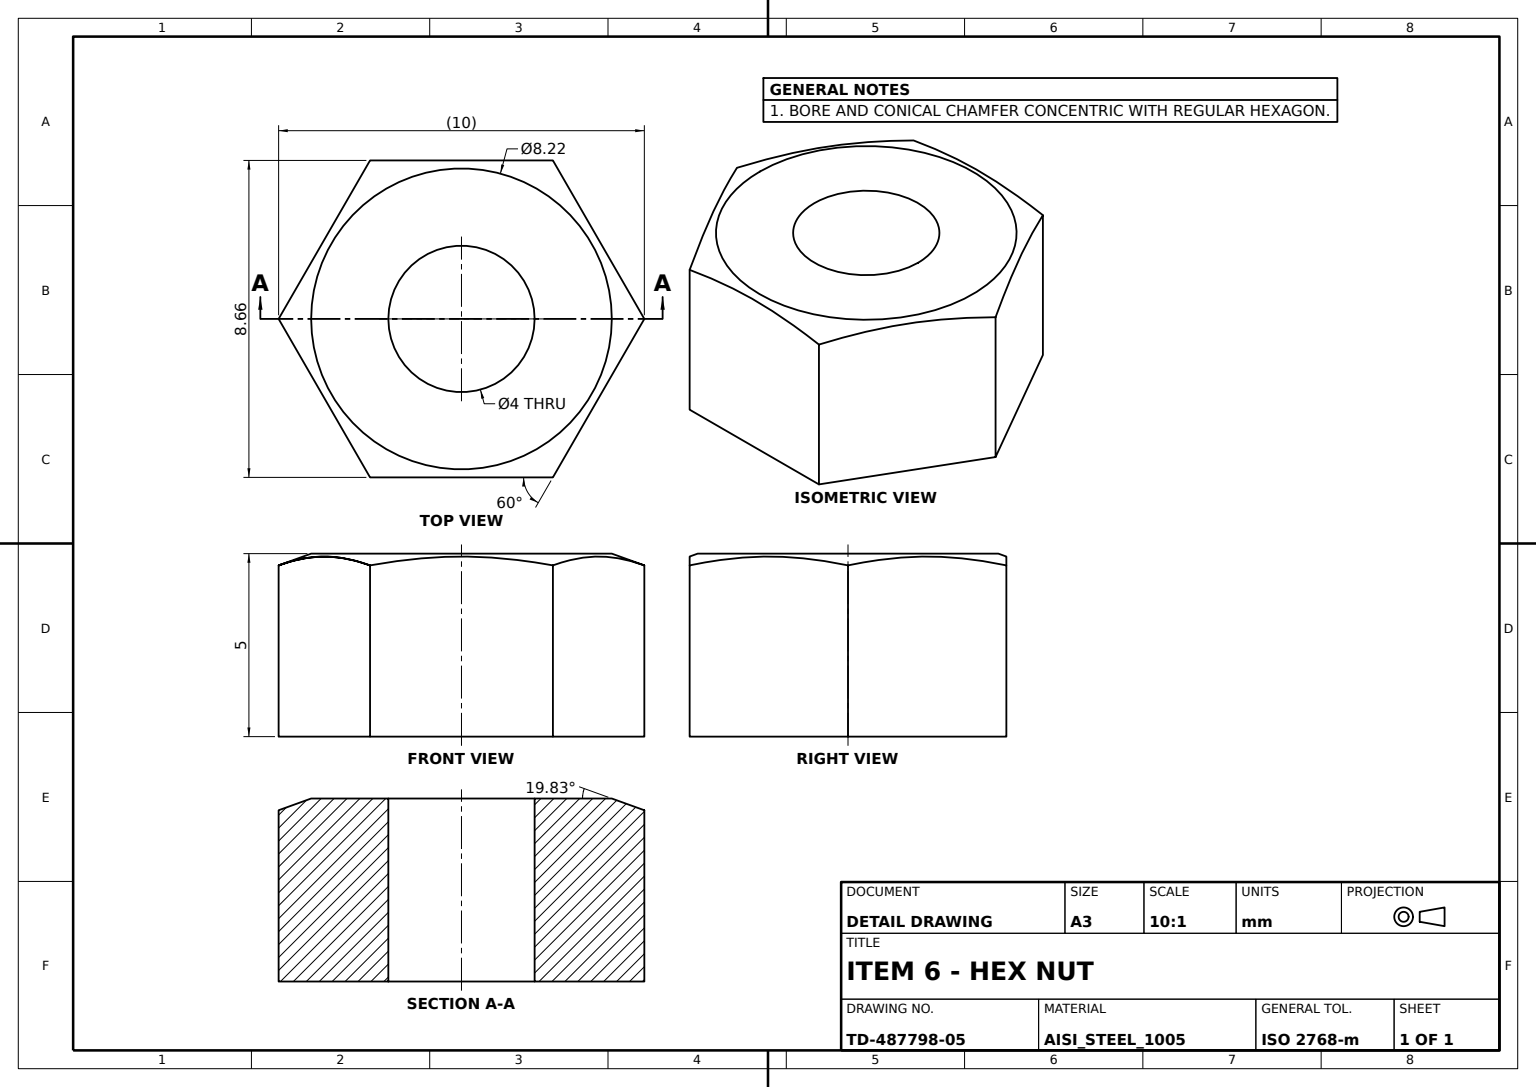
ISO-10303-21;
HEADER;
FILE_DESCRIPTION((''),'2;1');
FILE_NAME('','',(''),(''),'','','');
FILE_SCHEMA(('AUTOMOTIVE_DESIGN'));
ENDSEC;
DATA;
#1=APPLICATION_CONTEXT('');
#2=PRODUCT_CONTEXT('',#1,'mechanical');
#3=PRODUCT('','','',(#2));
#4=PRODUCT_DEFINITION_FORMATION('','',#3);
#5=PRODUCT_DEFINITION_CONTEXT('',#1,'design');
#6=PRODUCT_DEFINITION('','',#4,#5);
#7=PRODUCT_DEFINITION_SHAPE('','',#6);
#8=(LENGTH_UNIT()NAMED_UNIT(*)SI_UNIT(.MILLI.,.METRE.));
#9=(NAMED_UNIT(*)PLANE_ANGLE_UNIT()SI_UNIT($,.RADIAN.));
#10=(NAMED_UNIT(*)SI_UNIT($,.STERADIAN.)SOLID_ANGLE_UNIT());
#11=UNCERTAINTY_MEASURE_WITH_UNIT(LENGTH_MEASURE(0.005),#8,'distance_accuracy_value','');
#12=(GEOMETRIC_REPRESENTATION_CONTEXT(3)GLOBAL_UNCERTAINTY_ASSIGNED_CONTEXT((#11))GLOBAL_UNIT_ASSIGNED_CONTEXT((#8,#9,#10))REPRESENTATION_CONTEXT('',''));
#13=CARTESIAN_POINT('',(-2.5,-4.330127,4.679253));
#14=VERTEX_POINT('',#13);
#15=CARTESIAN_POINT('',(-5.,0.,4.679253));
#16=VERTEX_POINT('',#15);
#17=CARTESIAN_POINT('',(-2.916667,-3.608439,4.829483));
#18=CARTESIAN_POINT('',(-3.75,-2.165064,5.012071));
#19=CARTESIAN_POINT('',(-4.583333,-0.721688,4.829483));
#20=B_SPLINE_CURVE_WITH_KNOTS('',3,(#13,#17,#18,#19,#15),.UNSPECIFIED.,.F.,.F.,(4,1,4),(0.000000231,0.002500231,0.005000231),.UNSPECIFIED.);
#21=EDGE_CURVE('',#14,#16,#20,.T.);
#22=ORIENTED_EDGE('',*,*,#21,.T.);
#23=CARTESIAN_POINT('',(-5.,0.,0.));
#24=VERTEX_POINT('',#23);
#25=CARTESIAN_POINT('',(-5.,0.,5.));
#26=DIRECTION('',(0.,0.,-1.));
#27=VECTOR('',#26,1000.);
#28=LINE('',#25,#27);
#29=EDGE_CURVE('',#16,#24,#28,.T.);
#30=ORIENTED_EDGE('',*,*,#29,.T.);
#31=CARTESIAN_POINT('',(-2.5,-4.330127,0.));
#32=VERTEX_POINT('',#31);
#33=DIRECTION('',(0.5,-0.866025404,0.));
#34=VECTOR('',#33,1000.);
#35=LINE('',#23,#34);
#36=EDGE_CURVE('',#24,#32,#35,.T.);
#37=ORIENTED_EDGE('',*,*,#36,.T.);
#38=CARTESIAN_POINT('',(-2.5,-4.330127,5.));
#39=LINE('',#38,#27);
#40=EDGE_CURVE('',#14,#32,#39,.T.);
#41=ORIENTED_EDGE('',*,*,#40,.F.);
#42=EDGE_LOOP('',(#22,#30,#37,#41));
#43=FACE_BOUND('',#42,.T.);
#44=DIRECTION('',(0.866025404,0.5,0.));
#45=DIRECTION('',(-0.5,0.866025404,0.));
#46=AXIS2_PLACEMENT_3D('',#25,#44,#45);
#47=PLANE('',#46);
#48=ADVANCED_FACE('',(#43),#47,.F.);
#49=CARTESIAN_POINT('',(2.,0.,0.));
#50=VERTEX_POINT('',#49);
#51=CARTESIAN_POINT('',(0.,0.,0.));
#52=DIRECTION('',(1.,0.,0.));
#53=AXIS2_PLACEMENT_3D('',#51,#26,#52);
#54=CIRCLE('',#53,2.);
#55=EDGE_CURVE('',#50,#50,#54,.T.);
#56=ORIENTED_EDGE('',*,*,#55,.T.);
#57=EDGE_LOOP('',(#56));
#58=FACE_BOUND('',#57,.T.);
#59=CARTESIAN_POINT('',(2.,0.,5.));
#60=VERTEX_POINT('',#59);
#61=CARTESIAN_POINT('',(0.,0.,5.));
#62=AXIS2_PLACEMENT_3D('',#61,#26,#52);
#63=CIRCLE('',#62,2.);
#64=EDGE_CURVE('',#60,#60,#63,.T.);
#65=ORIENTED_EDGE('',*,*,#64,.F.);
#66=EDGE_LOOP('',(#65));
#67=FACE_BOUND('',#66,.T.);
#68=DIRECTION('',(0.,0.,1.));
#69=AXIS2_PLACEMENT_3D('',#51,#68,#52);
#70=CYLINDRICAL_SURFACE('',#69,2.);
#71=ADVANCED_FACE('',(#58,#67),#70,.F.);
#72=CARTESIAN_POINT('',(5.,0.,4.679253));
#73=VERTEX_POINT('',#72);
#74=CARTESIAN_POINT('',(5.,0.,0.));
#75=VERTEX_POINT('',#74);
#76=CARTESIAN_POINT('',(5.,0.,5.));
#77=LINE('',#76,#27);
#78=EDGE_CURVE('',#73,#75,#77,.T.);
#79=ORIENTED_EDGE('',*,*,#78,.F.);
#80=CARTESIAN_POINT('',(2.5,-4.330127,4.679253));
#81=VERTEX_POINT('',#80);
#82=CARTESIAN_POINT('',(4.583333,-0.721688,4.829483));
#83=CARTESIAN_POINT('',(3.75,-2.165064,5.012071));
#84=CARTESIAN_POINT('',(2.916667,-3.608439,4.829483));
#85=B_SPLINE_CURVE_WITH_KNOTS('',3,(#72,#82,#83,#84,#80),.UNSPECIFIED.,.F.,.F.,(4,1,4),(0.000000231,0.002500231,0.005000231),.UNSPECIFIED.);
#86=EDGE_CURVE('',#73,#81,#85,.T.);
#87=ORIENTED_EDGE('',*,*,#86,.T.);
#88=CARTESIAN_POINT('',(2.5,-4.330127,0.));
#89=VERTEX_POINT('',#88);
#90=CARTESIAN_POINT('',(2.5,-4.330127,5.));
#91=LINE('',#90,#27);
#92=EDGE_CURVE('',#81,#89,#91,.T.);
#93=ORIENTED_EDGE('',*,*,#92,.T.);
#94=DIRECTION('',(0.5,0.866025404,0.));
#95=VECTOR('',#94,1000.);
#96=LINE('',#88,#95);
#97=EDGE_CURVE('',#89,#75,#96,.T.);
#98=ORIENTED_EDGE('',*,*,#97,.T.);
#99=EDGE_LOOP('',(#79,#87,#93,#98));
#100=FACE_BOUND('',#99,.T.);
#101=DIRECTION('',(-0.866025404,0.5,0.));
#102=DIRECTION('',(-0.5,-0.866025404,0.));
#103=AXIS2_PLACEMENT_3D('',#90,#101,#102);
#104=PLANE('',#103);
#105=ADVANCED_FACE('',(#100),#104,.F.);
#106=CARTESIAN_POINT('',(2.5,4.330127,4.679253));
#107=VERTEX_POINT('',#106);
#108=CARTESIAN_POINT('',(2.916667,3.608439,4.829483));
#109=CARTESIAN_POINT('',(3.75,2.165064,5.012071));
#110=CARTESIAN_POINT('',(4.583333,0.721688,4.829483));
#111=B_SPLINE_CURVE_WITH_KNOTS('',3,(#106,#108,#109,#110,#72),.UNSPECIFIED.,.F.,.F.,(4,1,4),(0.000000231,0.002500231,0.005000231),.UNSPECIFIED.);
#112=EDGE_CURVE('',#107,#73,#111,.T.);
#113=ORIENTED_EDGE('',*,*,#112,.T.);
#114=ORIENTED_EDGE('',*,*,#78,.T.);
#115=CARTESIAN_POINT('',(2.5,4.330127,0.));
#116=VERTEX_POINT('',#115);
#117=VECTOR('',#45,1000.);
#118=LINE('',#74,#117);
#119=EDGE_CURVE('',#75,#116,#118,.T.);
#120=ORIENTED_EDGE('',*,*,#119,.T.);
#121=CARTESIAN_POINT('',(2.5,4.330127,5.));
#122=LINE('',#121,#27);
#123=EDGE_CURVE('',#107,#116,#122,.T.);
#124=ORIENTED_EDGE('',*,*,#123,.F.);
#125=EDGE_LOOP('',(#113,#114,#120,#124));
#126=FACE_BOUND('',#125,.T.);
#127=DIRECTION('',(-0.866025404,-0.5,0.));
#128=AXIS2_PLACEMENT_3D('',#76,#127,#33);
#129=PLANE('',#128);
#130=ADVANCED_FACE('',(#126),#129,.F.);
#131=ORIENTED_EDGE('',*,*,#29,.F.);
#132=CARTESIAN_POINT('',(-2.5,4.330127,4.679253));
#133=VERTEX_POINT('',#132);
#134=CARTESIAN_POINT('',(-4.583333,0.721688,4.829483));
#135=CARTESIAN_POINT('',(-3.75,2.165064,5.012071));
#136=CARTESIAN_POINT('',(-2.916667,3.608439,4.829483));
#137=B_SPLINE_CURVE_WITH_KNOTS('',3,(#15,#134,#135,#136,#132),.UNSPECIFIED.,.F.,.F.,(4,1,4),(0.000000231,0.002500231,0.005000231),.UNSPECIFIED.);
#138=EDGE_CURVE('',#16,#133,#137,.T.);
#139=ORIENTED_EDGE('',*,*,#138,.T.);
#140=CARTESIAN_POINT('',(-2.5,4.330127,0.));
#141=VERTEX_POINT('',#140);
#142=CARTESIAN_POINT('',(-2.5,4.330127,5.));
#143=LINE('',#142,#27);
#144=EDGE_CURVE('',#133,#141,#143,.T.);
#145=ORIENTED_EDGE('',*,*,#144,.T.);
#146=VECTOR('',#102,1000.);
#147=LINE('',#140,#146);
#148=EDGE_CURVE('',#141,#24,#147,.T.);
#149=ORIENTED_EDGE('',*,*,#148,.T.);
#150=EDGE_LOOP('',(#131,#139,#145,#149));
#151=FACE_BOUND('',#150,.T.);
#152=DIRECTION('',(0.866025404,-0.5,0.));
#153=AXIS2_PLACEMENT_3D('',#142,#152,#94);
#154=PLANE('',#153);
#155=ADVANCED_FACE('',(#151),#154,.F.);
#156=ORIENTED_EDGE('',*,*,#55,.F.);
#157=EDGE_LOOP('',(#156));
#158=FACE_BOUND('',#157,.T.);
#159=ORIENTED_EDGE('',*,*,#36,.F.);
#160=ORIENTED_EDGE('',*,*,#148,.F.);
#161=DIRECTION('',(-1.,0.,0.));
#162=VECTOR('',#161,1000.);
#163=LINE('',#115,#162);
#164=EDGE_CURVE('',#116,#141,#163,.T.);
#165=ORIENTED_EDGE('',*,*,#164,.F.);
#166=ORIENTED_EDGE('',*,*,#119,.F.);
#167=ORIENTED_EDGE('',*,*,#97,.F.);
#168=VECTOR('',#52,1000.);
#169=LINE('',#31,#168);
#170=EDGE_CURVE('',#32,#89,#169,.T.);
#171=ORIENTED_EDGE('',*,*,#170,.F.);
#172=EDGE_LOOP('',(#159,#160,#165,#166,#167,#171));
#173=FACE_BOUND('',#172,.T.);
#174=PLANE('',#69);
#175=ADVANCED_FACE('',(#158,#173),#174,.F.);
#176=ORIENTED_EDGE('',*,*,#92,.F.);
#177=CARTESIAN_POINT('',(-1.670728,-4.330127,4.828751));
#178=CARTESIAN_POINT('',(0.008278,-4.330127,5.012718));
#179=CARTESIAN_POINT('',(1.669804,-4.330127,4.828917));
#180=B_SPLINE_CURVE_WITH_KNOTS('',3,(#13,#177,#178,#179,#80),.UNSPECIFIED.,.F.,.F.,(4,1,4),(0.004242185,0.006765661,0.009289136),.UNSPECIFIED.);
#181=EDGE_CURVE('',#81,#14,#180,.F.);
#182=ORIENTED_EDGE('',*,*,#181,.T.);
#183=ORIENTED_EDGE('',*,*,#40,.T.);
#184=ORIENTED_EDGE('',*,*,#170,.T.);
#185=EDGE_LOOP('',(#176,#182,#183,#184));
#186=FACE_BOUND('',#185,.T.);
#187=DIRECTION('',(0.,1.,0.));
#188=AXIS2_PLACEMENT_3D('',#38,#187,#68);
#189=PLANE('',#188);
#190=ADVANCED_FACE('',(#186),#189,.F.);
#191=CARTESIAN_POINT('',(-4.110399,0.,5.));
#192=VERTEX_POINT('',#191);
#193=AXIS2_PLACEMENT_3D('',#61,#26,#161);
#194=CIRCLE('',#193,4.110399);
#195=EDGE_CURVE('',#192,#192,#194,.T.);
#196=ORIENTED_EDGE('',*,*,#195,.T.);
#197=EDGE_LOOP('',(#196));
#198=FACE_BOUND('',#197,.T.);
#199=ORIENTED_EDGE('',*,*,#86,.F.);
#200=ORIENTED_EDGE('',*,*,#112,.F.);
#201=CARTESIAN_POINT('',(-1.670728,4.330127,4.828751));
#202=CARTESIAN_POINT('',(0.008278,4.330127,5.012718));
#203=CARTESIAN_POINT('',(1.669804,4.330127,4.828917));
#204=B_SPLINE_CURVE_WITH_KNOTS('',3,(#132,#201,#202,#203,#106),.UNSPECIFIED.,.F.,.F.,(4,1,4),(0.004242185,0.006765661,0.009289136),.UNSPECIFIED.);
#205=EDGE_CURVE('',#133,#107,#204,.T.);
#206=ORIENTED_EDGE('',*,*,#205,.F.);
#207=ORIENTED_EDGE('',*,*,#138,.F.);
#208=ORIENTED_EDGE('',*,*,#21,.F.);
#209=ORIENTED_EDGE('',*,*,#181,.F.);
#210=EDGE_LOOP('',(#199,#200,#206,#207,#208,#209));
#211=FACE_BOUND('',#210,.T.);
#212=CONICAL_SURFACE('',#193,4.110398709,1.224752534);
#213=ADVANCED_FACE('',(#198,#211),#212,.T.);
#214=ORIENTED_EDGE('',*,*,#144,.F.);
#215=ORIENTED_EDGE('',*,*,#205,.T.);
#216=ORIENTED_EDGE('',*,*,#123,.T.);
#217=ORIENTED_EDGE('',*,*,#164,.T.);
#218=EDGE_LOOP('',(#214,#215,#216,#217));
#219=FACE_BOUND('',#218,.T.);
#220=DIRECTION('',(0.,-1.,0.));
#221=AXIS2_PLACEMENT_3D('',#121,#220,#26);
#222=PLANE('',#221);
#223=ADVANCED_FACE('',(#219),#222,.F.);
#224=ORIENTED_EDGE('',*,*,#195,.F.);
#225=EDGE_LOOP('',(#224));
#226=FACE_BOUND('',#225,.T.);
#227=ORIENTED_EDGE('',*,*,#64,.T.);
#228=EDGE_LOOP('',(#227));
#229=FACE_BOUND('',#228,.T.);
#230=AXIS2_PLACEMENT_3D('',#61,#68,#52);
#231=PLANE('',#230);
#232=ADVANCED_FACE('',(#226,#229),#231,.T.);
#233=CLOSED_SHELL('',(#48,#71,#105,#130,#155,#175,#190,#213,#223,#232));
#234=MANIFOLD_SOLID_BREP('',#233);
#235=ADVANCED_BREP_SHAPE_REPRESENTATION('',(#234),#12);
#236=SHAPE_DEFINITION_REPRESENTATION(#7,#235);
ENDSEC;
END-ISO-10303-21;
